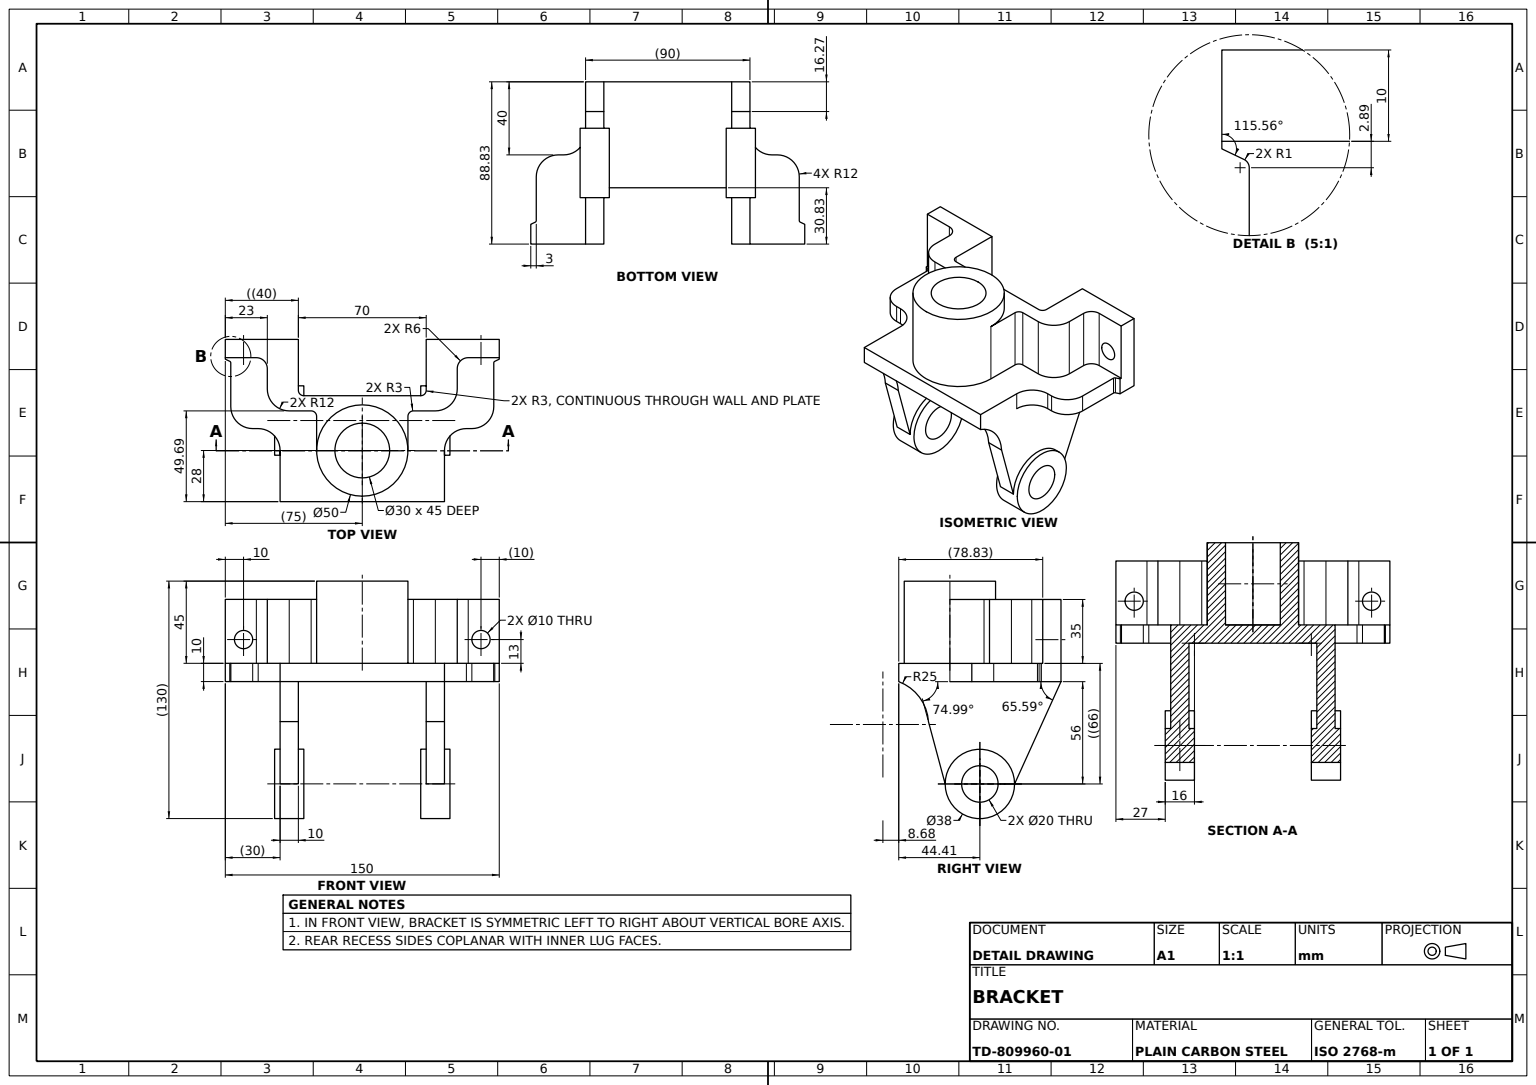
solid
v1 (-45,-61,-25.413573)
v2 (-45,-26.908854,-16.270281)
e1 v1 v2 LINE
v3 (-45,-5,0)
e2 v2 v3 CIRCLE(AX(P(-45,-28.443833,8.682552),D(1,0,0),D(0,0,1)),25)
v4 (-45,5,0)
e3 v4 v3 LINE
v5 (-45,5,-28)
e4 v5 v4 LINE
v6 (-45,-5,-28)
e5 v5 v6 LINE
v7 (-45,-5,-88.827146)
e6 v7 v6 LINE
v8 (-45,-61,-63.413573)
e7 v8 v7 LINE
e8 v1 v8 CIRCLE(AX(P(-45,-61,-44.413573),D(-1,0,0),D(0,0,1)),19)
face PLANE(AX(P(-45,5,0),D(1,0,0),D(0,0,-1))) rev [e1 e2 -e3 -e4 e5 -e6 -e7 -e8]
v9 (45,-5,-28)
v10 (57,-5,-40)
e9 v9 v10 CIRCLE(AX(P(57,-5,-28),D(0,-1,0),D(0,0,1)),12)
v11 (57,5,-40)
e10 v11 v10 LINE
v12 (45,5,-28)
e11 v12 v11 CIRCLE(AX(P(57,5,-28),D(0,-1,0),D(0,0,1)),12)
e12 v12 v9 LINE
face CYL(AX(P(57,5,-28),D(0,-1,0),D(0,0,-1)),12) rev [e9 -e10 -e11 e12]
v13 (35,-61,-63.413573)
v14 (32,-61,-63.413573)
e13 v13 v14 LINE
v15 (32,-61,-25.413573)
e14 v15 v14 CIRCLE(AX(P(32,-61,-44.413573),D(-1,0,0),D(0,0,1)),19)
v16 (35,-61,-25.413573)
e15 v16 v15 LINE
e16 v16 v13 CIRCLE(AX(P(35,-61,-44.413573),D(-1,0,0),D(0,0,1)),19)
face CYL(AX(P(48,-61,-44.413573),D(-1,0,0),D(0,0,1)),19) [e13 -e14 -e15 e16]
v17 (-32,-61,-34.413573)
v18 (-32,-61,-54.413573)
e17 v17 v18 CIRCLE(AX(P(-32,-61,-44.413573),D(-1,0,0),D(0,0,1)),10)
e18 v18 v17 CIRCLE(AX(P(-32,-61,-44.413573),D(-1,0,0),D(0,0,1)),10)
v19 (-32,-61,-63.413573)
v20 (-32,-61,-25.413573)
e19 v19 v20 CIRCLE(AX(P(-32,-61,-44.413573),D(-1,0,0),D(0,0,1)),19)
e20 v20 v19 CIRCLE(AX(P(-32,-61,-44.413573),D(-1,0,0),D(0,0,1)),19)
face PLANE(AX(P(-32,-61,-44.413573),D(-1,0,0),D(0,0,1))) rev [e17 e18] [-e19 -e20]
v21 (60,5,-40)
e21 v11 v21 LINE
v22 (60,-5,-40)
e22 v10 v22 LINE
e23 v21 v22 LINE
face PLANE(AX(P(57,5,-40),D(0,0,-1),D(-1,0,0))) rev [-e21 e10 e22 -e23]
v23 (-48,-61,-34.413573)
e24 v23 v17 LINE
v24 (-48,-61,-54.413573)
e25 v23 v24 CIRCLE(AX(P(-48,-61,-44.413573),D(-1,0,0),D(0,0,1)),10)
e26 v24 v18 LINE
face CYL(AX(P(-48,-61,-44.413573),D(1,0,0),D(0,0,-1)),10) rev [-e24 e25 e26 -e17]
v25 (35,-5,-61)
v26 (35,-5,0)
e27 v25 v26 LINE
v27 (-35,-5,0)
e28 v27 v26 LINE
v28 (-35,-5,-61)
e29 v28 v27 LINE
v29 (-32,-5,-58)
e30 v29 v28 CIRCLE(AX(P(-32,-5,-61),D(0,-1,0),D(0,0,1)),3)
v30 (32,-5,-58)
e31 v30 v29 LINE
e32 v25 v30 CIRCLE(AX(P(32,-5,-61),D(0,-1,0),D(0,0,1)),3)
face PLANE(AX(P(-57,-5,-28),D(0,-1,0),D(0,0,-1))) [e27 -e28 -e29 -e30 -e31 -e32]
v31 (-28,40,-49.686128)
v32 (-28,5,-49.686128)
e33 v31 v32 LINE
v33 (-25,5,-46.686128)
e34 v32 v33 CIRCLE(AX(P(-28,5,-46.686128),D(0,-1,0),D(0,0,1)),3)
v34 (-25,40,-46.686128)
e35 v34 v33 LINE
e36 v31 v34 CIRCLE(AX(P(-28,40,-46.686128),D(0,-1,0),D(0,0,1)),3)
face CYL(AX(P(-28,40,-46.686128),D(0,-1,0),D(0,0,-1)),3) rev [e33 e34 -e35 -e36]
v35 (-70,18,-78.827146)
v36 (-70,18,-88.827146)
e37 v35 v36 LINE
v37 (-60,18,-88.827146)
e38 v36 v37 CIRCLE(AX(P(-65,18,-88.827146),D(0,0,-1),D(-1,0,0)),5)
v38 (-60,18,-78.827146)
e39 v38 v37 LINE
e40 v35 v38 CIRCLE(AX(P(-65,18,-78.827146),D(0,0,-1),D(-1,0,0)),5)
face CYL(AX(P(-65,18,-66.327146),D(0,0,-1),D(-1,0,0)),5) rev [e37 e38 -e39 -e40]
v39 (52,40,-61.686128)
v40 (52,5,-61.686128)
e41 v39 v40 LINE
v41 (52,5,-72.827146)
e42 v41 v40 LINE
v42 (52,40,-72.827146)
e43 v42 v41 LINE
e44 v42 v39 LINE
face PLANE(AX(P(52,40,0),D(1,0,0),D(0,0,-1))) [e41 -e42 -e43 e44]
e45 v24 v23 CIRCLE(AX(P(-48,-61,-44.413573),D(-1,0,0),D(0,0,1)),10)
v43 (-48,-61,-63.413573)
v44 (-48,-61,-25.413573)
e46 v43 v44 CIRCLE(AX(P(-48,-61,-44.413573),D(-1,0,0),D(0,0,1)),19)
e47 v44 v43 CIRCLE(AX(P(-48,-61,-44.413573),D(-1,0,0),D(0,0,1)),19)
face PLANE(AX(P(-48,-61,-44.413573),D(-1,0,0),D(0,0,1))) [-e45 -e25] [e46 e47]
v45 (0,50,-43)
v46 (0,50,-13)
e48 v45 v46 CIRCLE(AX(P(0,50,-28),D(0,1,0),D(0,0,1)),15)
v47 (0,5,-13)
e49 v46 v47 LINE
v48 (0,5,-43)
e50 v48 v47 CIRCLE(AX(P(0,5,-28),D(0,1,0),D(0,0,1)),15)
e51 v45 v48 LINE
face CYL(AX(P(0,50,-28),D(0,-1,0),D(0,0,-1)),15) rev [e48 e49 -e50 -e51]
v49 (60,18,-88.827146)
v50 (70,18,-88.827146)
e52 v49 v50 CIRCLE(AX(P(65,18,-88.827146),D(0,0,-1),D(-1,0,0)),5)
v51 (70,18,-78.827146)
e53 v51 v50 LINE
v52 (60,18,-78.827146)
e54 v51 v52 CIRCLE(AX(P(65,18,-78.827146),D(0,0,1),D(1,0,0)),5)
e55 v52 v49 LINE
face CYL(AX(P(65,18,-66.327146),D(0,0,-1),D(-1,0,0)),5) rev [e52 -e53 e54 e55]
v53 (75,-5,-88.827146)
v54 (45,-5,-88.827146)
e56 v53 v54 LINE
v55 (35,-5,-88.827146)
e57 v55 v54 LINE
v56 (35,40,-88.827146)
e58 v55 v56 LINE
v57 (75,40,-88.827146)
e59 v57 v56 LINE
e60 v53 v57 LINE
e61 v50 v49 CIRCLE(AX(P(65,18,-88.827146),D(0,0,-1),D(-1,0,0)),5)
face PLANE(AX(P(35,-5,-88.827146),D(0,0,-1),D(-1,0,0))) [e56 -e57 e58 -e59 -e60] [-e61 -e52]
e62 v14 v15 CIRCLE(AX(P(32,-61,-44.413573),D(-1,0,0),D(0,0,1)),19)
v58 (45,-61,-63.413573)
e63 v13 v58 LINE
v59 (48,-61,-63.413573)
e64 v59 v58 LINE
v60 (48,-61,-25.413573)
e65 v59 v60 CIRCLE(AX(P(48,-61,-44.413573),D(-1,0,0),D(0,0,1)),19)
v61 (45,-61,-25.413573)
e66 v60 v61 LINE
e67 v16 v61 LINE
face CYL(AX(P(48,-61,-44.413573),D(-1,0,0),D(0,0,1)),19) [e15 -e62 -e13 e63 -e64 e65 e66 -e67]
e68 v58 v54 LINE
e69 v13 v55 LINE
face PLANE(AX(P(35,-34.280712,-75.539155),D(0,-0.413250701,-0.910617295),D(0,0.910617295,-0.413250701))) [-e68 -e63 e69 e57]
v62 (-72,5,-52)
v63 (-60,5,-40)
e70 v62 v63 CIRCLE(AX(P(-60,5,-52),D(0,1,0),D(0,0,-1)),12)
v64 (-72,-5,-52)
e71 v62 v64 LINE
v65 (-60,-5,-40)
e72 v64 v65 CIRCLE(AX(P(-60,-5,-52),D(0,1,0),D(0,0,-1)),12)
e73 v63 v65 LINE
face CYL(AX(P(-60,5,-52),D(0,-1,0),D(0,0,-1)),12) [-e70 e71 e72 -e73]
v66 (40,40,-49.686128)
v67 (40,5,-49.686128)
e74 v66 v67 LINE
e75 v40 v67 CIRCLE(AX(P(40,5,-61.686128),D(0,-1,0),D(0,0,1)),12)
e76 v39 v66 CIRCLE(AX(P(40,40,-61.686128),D(0,-1,0),D(0,0,1)),12)
face CYL(AX(P(40,40,-61.686128),D(0,-1,0),D(0,0,-1)),12) [e74 -e75 -e41 e76]
v68 (32,40,-58)
v69 (-32,40,-58)
e77 v68 v69 LINE
e78 v68 v30 LINE
e79 v69 v29 LINE
face PLANE(AX(P(-32,5,-58),D(0,0,1),D(1,0,0))) rev [-e77 e78 e31 -e79]
v70 (45,5,0)
e80 v70 v12 LINE
v71 (45,-5,0)
e81 v70 v71 LINE
v72 (45,-26.908854,-16.270281)
e82 v72 v71 CIRCLE(AX(P(45,-28.443833,8.682552),D(1,0,0),D(0,0,1)),25)
e83 v61 v72 LINE
e84 v61 v58 CIRCLE(AX(P(45,-61,-44.413573),D(-1,0,0),D(0,0,1)),19)
e85 v54 v9 LINE
face PLANE(AX(P(45,5,0),D(-1,0,0),D(0,0,1))) rev [-e80 e81 -e82 -e83 e84 e68 e85 -e12]
v73 (35,40,-61)
e86 v73 v68 CIRCLE(AX(P(32,40,-61),D(0,-1,0),D(0,0,1)),3)
e87 v73 v25 LINE
face CYL(AX(P(32,5,-61),D(0,-1,0),D(0,0,-1)),3) rev [e32 -e78 -e86 e87]
v74 (25,40,-28)
v75 (25,40,-46.686128)
e88 v74 v75 LINE
v76 (25,5,-28)
e89 v74 v76 LINE
v77 (25,5,-46.686128)
e90 v76 v77 LINE
e91 v75 v77 LINE
face PLANE(AX(P(25,40,0),D(-1,0,0),D(0,0,1))) rev [-e88 e89 e90 -e91]
e92 v44 v1 LINE
e93 v43 v8 LINE
face CYL(AX(P(-48,-61,-44.413573),D(1,0,0),D(0,0,-1)),19) [e92 e8 -e93 -e47]
v78 (72,5,-52)
e94 v21 v78 CIRCLE(AX(P(60,5,-52),D(0,1,0),D(0,0,-1)),12)
v79 (72,-5,-52)
e95 v22 v79 CIRCLE(AX(P(60,-5,-52),D(0,1,0),D(0,0,-1)),12)
e96 v78 v79 LINE
face CYL(AX(P(60,5,-52),D(0,-1,0),D(0,0,-1)),12) [-e94 e23 e95 -e96]
v80 (-52,40,-72.827146)
v81 (-58,40,-78.827146)
e97 v80 v81 CIRCLE(AX(P(-58,40,-72.827146),D(0,1,0),D(0,0,1)),6)
v82 (-58,5,-78.827146)
e98 v81 v82 LINE
v83 (-52,5,-72.827146)
e99 v83 v82 CIRCLE(AX(P(-58,5,-72.827146),D(0,1,0),D(0,0,1)),6)
e100 v80 v83 LINE
face CYL(AX(P(-58,40,-72.827146),D(0,-1,0),D(0,0,-1)),6) rev [e97 e98 -e99 -e100]
e101 v3 v27 LINE
e102 v26 v71 LINE
e103 v4 v70 LINE
face PLANE(AX(P(-45,5,0),D(0,0,-1),D(-1,0,0))) rev [e101 e28 e102 -e81 -e103 e3]
v84 (-35,-5,-88.827146)
v85 (-35,40,-88.827146)
e104 v84 v85 LINE
e105 v84 v7 LINE
v86 (-75,-5,-88.827146)
e106 v7 v86 LINE
v87 (-75,40,-88.827146)
e107 v86 v87 LINE
e108 v85 v87 LINE
e109 v37 v36 CIRCLE(AX(P(-65,18,-88.827146),D(0,0,-1),D(-1,0,0)),5)
face PLANE(AX(P(-75,-5,-88.827146),D(0,0,-1),D(-1,0,0))) [-e104 e105 e106 e107 -e108] [-e38 -e109]
v88 (72,5,-75.935047)
v89 (72,-5,-75.935047)
e110 v88 v89 LINE
v90 (72.56856,-5,-76.837188)
e111 v89 v90 CIRCLE(AX(P(73,-5,-75.935047),D(0,-1,0),D(0,0,1)),1)
v91 (72.56856,5,-76.837188)
e112 v91 v90 LINE
e113 v88 v91 CIRCLE(AX(P(73,5,-75.935047),D(0,-1,0),D(0,0,1)),1)
face CYL(AX(P(73,5,-75.935047),D(0,-1,0),D(0,0,-1)),1) rev [e110 e111 -e112 -e113]
face CYL(AX(P(-48,-61,-44.413573),D(1,0,0),D(0,0,-1)),10) rev [-e18 -e26 e45 e24]
v92 (-72.56856,5,-76.837188)
v93 (-72.56856,-5,-76.837188)
e114 v92 v93 LINE
v94 (-72,-5,-75.935047)
e115 v93 v94 CIRCLE(AX(P(-73,-5,-75.935047),D(0,-1,0),D(0,0,1)),1)
v95 (-72,5,-75.935047)
e116 v95 v94 LINE
e117 v92 v95 CIRCLE(AX(P(-73,5,-75.935047),D(0,-1,0),D(0,0,1)),1)
face CYL(AX(P(-73,5,-75.935047),D(0,-1,0),D(0,0,-1)),1) rev [e114 e115 -e116 -e117]
e118 v60 v59 CIRCLE(AX(P(48,-61,-44.413573),D(-1,0,0),D(0,0,1)),19)
face CYL(AX(P(48,-61,-44.413573),D(-1,0,0),D(0,0,1)),19) [e118 e64 -e84 -e66]
e119 v38 v35 CIRCLE(AX(P(-65,18,-78.827146),D(0,0,-1),D(-1,0,0)),5)
v96 (-75,5,-78.827146)
e120 v96 v82 LINE
v97 (-75,40,-78.827146)
e121 v97 v81 LINE
e122 v97 v96 LINE
face PLANE(AX(P(0,40,-78.827146),D(0,0,-1),D(-1,0,0))) rev [e119 e40] [e120 -e98 -e121 e122]
face CYL(AX(P(-65,18,-66.327146),D(0,0,-1),D(-1,0,0)),5) rev [e109 -e37 -e119 e39]
v98 (-25,5,-28)
e123 v98 v33 LINE
v99 (-25,40,-28)
e124 v99 v98 LINE
e125 v99 v34 LINE
face PLANE(AX(P(-25,40,0),D(-1,0,0),D(0,0,1))) [-e123 -e124 e125 e35]
v100 (58,40,-78.827146)
v101 (58,5,-78.827146)
e126 v100 v101 LINE
v102 (75,5,-78.827146)
e127 v102 v101 LINE
v103 (75,40,-78.827146)
e128 v103 v102 LINE
e129 v103 v100 LINE
e130 v52 v51 CIRCLE(AX(P(65,18,-78.827146),D(0,0,1),D(1,0,0)),5)
face PLANE(AX(P(0,40,-78.827146),D(0,0,1),D(1,0,0))) [e126 -e127 -e128 e129] [-e130 -e54]
v104 (-35,-26.908854,-16.270281)
e131 v104 v2 LINE
e132 v104 v27 CIRCLE(AX(P(-35,-28.443833,8.682552),D(1,0,0),D(0,0,1)),25)
face CYL(AX(P(-35,-28.443833,8.682552),D(-1,0,0),D(0,0,1)),25) rev [-e2 -e131 e132 -e101]
v105 (-57,5,-40)
e133 v105 v5 CIRCLE(AX(P(-57,5,-28),D(0,-1,0),D(0,0,-1)),12)
v106 (-57,-5,-40)
e134 v105 v106 LINE
e135 v106 v6 CIRCLE(AX(P(-57,-5,-28),D(0,-1,0),D(0,0,-1)),12)
face CYL(AX(P(-57,5,-28),D(0,-1,0),D(0,0,-1)),12) rev [-e133 e134 e135 -e5]
v107 (0,50,-3)
v108 (0,50,-53)
e136 v107 v108 CIRCLE(AX(P(0,50,-28),D(0,1,0),D(0,0,1)),25)
e137 v108 v107 CIRCLE(AX(P(0,50,-28),D(0,1,0),D(0,0,1)),25)
e138 v46 v45 CIRCLE(AX(P(0,50,-28),D(0,1,0),D(0,0,1)),15)
face PLANE(AX(P(0,50,0),D(0,1,0),D(0,0,1))) [e136 e137] [-e48 -e138]
v109 (28,40,-49.686128)
e139 v109 v66 LINE
v110 (28,5,-49.686128)
e140 v109 v110 LINE
e141 v110 v67 LINE
face PLANE(AX(P(0,40,-49.686128),D(0,0,-1),D(-1,0,0))) rev [-e139 e140 e141 -e74]
e142 v47 v48 CIRCLE(AX(P(0,5,-28),D(0,1,0),D(0,0,1)),15)
face PLANE(AX(P(-57,5,-28),D(0,-1,0),D(0,0,-1))) rev [e142 e50]
e143 v65 v106 LINE
e144 v63 v105 LINE
face PLANE(AX(P(-57,5,-40),D(0,0,-1),D(-1,0,0))) rev [e73 e143 -e134 -e144]
v111 (-35,-61,-63.413573)
e145 v111 v84 LINE
e146 v111 v8 LINE
face PLANE(AX(P(-35,-34.280712,-75.539155),D(0,0.413250701,0.910617295),D(0,-0.910617295,0.413250701))) rev [-e105 -e145 e146 e7]
v112 (-75,5,-78)
e147 v112 v92 LINE
v113 (-75,-5,-78)
e148 v112 v113 LINE
e149 v113 v93 LINE
face PLANE(AX(P(-75,5,-78),D(0.431440099,0,-0.902141586),D(-0.902141586,0,-0.431440099))) rev [-e114 -e147 e148 e149]
v114 (-40,40,-49.686128)
v115 (-40,5,-49.686128)
e150 v114 v115 LINE
e151 v32 v115 LINE
e152 v31 v114 LINE
face PLANE(AX(P(0,40,-49.686128),D(0,0,1),D(1,0,0))) [e150 -e151 -e33 e152]
face CYL(AX(P(0,50,-28),D(0,-1,0),D(0,0,-1)),15) rev [e138 e51 -e142 -e49]
v116 (48,-61,-34.413573)
v117 (48,-61,-54.413573)
e153 v116 v117 CIRCLE(AX(P(48,-61,-44.413573),D(-1,0,0),D(0,0,1)),10)
v118 (32,-61,-34.413573)
e154 v116 v118 LINE
v119 (32,-61,-54.413573)
e155 v118 v119 CIRCLE(AX(P(32,-61,-44.413573),D(-1,0,0),D(0,0,1)),10)
e156 v117 v119 LINE
face CYL(AX(P(48,-61,-44.413573),D(-1,0,0),D(0,0,1)),10) rev [-e153 e154 e155 -e156]
v120 (35,-26.908854,-16.270281)
e157 v120 v26 CIRCLE(AX(P(35,-28.443833,8.682552),D(1,0,0),D(0,0,1)),25)
e158 v120 v72 LINE
face CYL(AX(P(35,-28.443833,8.682552),D(1,0,0),D(0,0,-1)),25) rev [-e102 -e157 e158 e82]
e159 v119 v118 CIRCLE(AX(P(32,-61,-44.413573),D(-1,0,0),D(0,0,1)),10)
face PLANE(AX(P(32,-61,-44.413573),D(1,0,0),D(0,0,1))) rev [e62 e14] [-e159 -e155]
v121 (-35,-61,-25.413573)
e160 v121 v1 LINE
e161 v121 v104 LINE
face PLANE(AX(P(-35,2.265167,-8.445768),D(0,-0.259046303,0.965864904),D(0,-0.965864904,-0.259046303))) [e131 -e1 -e160 e161]
e162 v94 v64 LINE
e163 v86 v113 LINE
face PLANE(AX(P(-57,-5,-28),D(0,-1,0),D(0,0,-1))) [-e72 -e162 -e115 -e149 -e163 -e106 e6 -e135 -e143]
e164 v56 v73 LINE
e165 v16 v120 LINE
face PLANE(AX(P(35,5,-61),D(1,0,0),D(0,0,-1))) rev [-e164 -e58 -e69 -e16 e165 e157 -e27 -e87]
e166 v96 v112 LINE
e167 v87 v97 LINE
face PLANE(AX(P(-75,-5,-78),D(-1,0,0),D(0,0,1))) [-e107 e163 -e148 -e166 -e122 -e167]
e168 v121 v111 CIRCLE(AX(P(-35,-61,-44.413573),D(-1,0,0),D(0,0,1)),19)
v122 (-35,40,-61)
e169 v122 v85 LINE
e170 v122 v28 LINE
face PLANE(AX(P(-35,5,-78),D(-1,0,0),D(0,0,1))) rev [e29 -e132 -e161 e168 e145 e104 -e169 e170]
e171 v103 v57 LINE
v123 (75,5,-78)
e172 v123 v102 LINE
v124 (75,-5,-78)
e173 v123 v124 LINE
e174 v124 v53 LINE
face PLANE(AX(P(75,-5,-88.827146),D(1,0,0),D(0,0,-1))) [e60 -e171 e128 -e172 e173 e174]
v125 (0,40,-53)
e175 v108 v125 LINE
e176 v125 v99 CIRCLE(AX(P(0,40,-28),D(0,1,0),D(0,0,1)),25)
v126 (0,5,-3)
e177 v98 v126 CIRCLE(AX(P(0,5,-28),D(0,1,0),D(0,0,1)),25)
e178 v107 v126 LINE
face CYL(AX(P(0,50,-28),D(0,-1,0),D(0,0,-1)),25) [e175 e176 e124 e177 -e178 -e137]
e179 v117 v116 CIRCLE(AX(P(48,-61,-44.413573),D(-1,0,0),D(0,0,1)),10)
face PLANE(AX(P(48,-61,-44.413573),D(1,0,0),D(0,0,1))) [e179 e153] [-e118 -e65]
face PLANE(AX(P(35,2.265167,-8.445768),D(0,0.259046303,-0.965864904),D(0,0.965864904,0.259046303))) rev [e83 -e158 -e165 e67]
v127 (-52,40,-61.686128)
v128 (-52,5,-61.686128)
e180 v127 v128 LINE
e181 v80 v127 LINE
e182 v83 v128 LINE
face PLANE(AX(P(-52,40,0),D(1,0,0),D(0,0,-1))) rev [-e180 -e181 e100 e182]
e183 v69 v122 CIRCLE(AX(P(-32,40,-61),D(0,-1,0),D(0,0,1)),3)
face CYL(AX(P(-32,5,-61),D(0,-1,0),D(0,0,-1)),3) rev [e30 -e170 -e183 e79]
face CYL(AX(P(48,-61,-44.413573),D(-1,0,0),D(0,0,1)),10) rev [-e179 e156 e159 -e154]
e184 v110 v77 CIRCLE(AX(P(28,5,-46.686128),D(0,1,0),D(0,0,1)),3)
e185 v109 v75 CIRCLE(AX(P(28,40,-46.686128),D(0,1,0),D(0,0,1)),3)
face CYL(AX(P(28,40,-46.686128),D(0,-1,0),D(0,0,-1)),3) rev [e91 -e184 -e140 e185]
e186 v95 v62 LINE
face PLANE(AX(P(-72,5,-52),D(1,0,0),D(0,0,-1))) rev [e116 e162 -e71 -e186]
e187 v74 v125 CIRCLE(AX(P(0,40,-28),D(0,1,0),D(0,0,1)),25)
e188 v126 v76 CIRCLE(AX(P(0,5,-28),D(0,1,0),D(0,0,1)),25)
face CYL(AX(P(0,50,-28),D(0,-1,0),D(0,0,-1)),25) [e187 -e175 -e136 e178 e188 -e89]
e189 v79 v89 LINE
e190 v78 v88 LINE
face PLANE(AX(P(72,5,-52),D(-1,0,0),D(0,0,1))) rev [e189 -e110 -e190 e96]
e191 v121 v20 LINE
e192 v111 v19 LINE
face CYL(AX(P(-48,-61,-44.413573),D(1,0,0),D(0,0,-1)),19) [e19 -e191 e160 -e92 -e46 e93 -e146 e192]
e193 v114 v127 CIRCLE(AX(P(-40,40,-61.686128),D(0,-1,0),D(0,0,1)),12)
e194 v42 v100 CIRCLE(AX(P(58,40,-72.827146),D(0,-1,0),D(0,0,1)),6)
face PLANE(AX(P(0,40,0),D(0,1,0),D(0,0,1))) [e169 e108 e167 e121 -e97 e181 -e193 -e152 e36 -e125 -e176 -e187 e88 -e185 e139 -e76 -e44 e194 -e129 e171 e59 e164 e86 e77 e183]
e195 v90 v124 LINE
e196 v91 v123 LINE
face PLANE(AX(P(75,5,-78),D(-0.431440099,0,-0.902141586),D(-0.902141586,0,0.431440099))) rev [e195 -e173 -e196 e112]
face CYL(AX(P(-48,-61,-44.413573),D(1,0,0),D(0,0,-1)),19) [-e192 -e168 e191 e20]
e197 v41 v101 CIRCLE(AX(P(58,5,-72.827146),D(0,-1,0),D(0,0,1)),6)
e198 v115 v128 CIRCLE(AX(P(-40,5,-61.686128),D(0,-1,0),D(0,0,1)),12)
face PLANE(AX(P(-57,5,-28),D(0,-1,0),D(0,0,-1))) rev [e186 e70 e144 e133 e4 e103 e80 e11 e21 e94 e190 e113 e196 e172 e127 -e197 e42 e75 -e141 e184 -e90 -e188 -e177 e123 -e34 e151 e198 -e182 e99 -e120 e166 e147 e117]
face CYL(AX(P(65,18,-66.327146),D(0,0,-1),D(-1,0,0)),5) rev [-e55 e130 e53 e61]
face CYL(AX(P(-40,40,-61.686128),D(0,-1,0),D(0,0,-1)),12) [e180 -e198 -e150 e193]
face PLANE(AX(P(-57,-5,-28),D(0,-1,0),D(0,0,-1))) [-e189 -e95 -e22 -e9 -e85 -e56 -e174 -e195 -e111]
face CYL(AX(P(58,40,-72.827146),D(0,-1,0),D(0,0,-1)),6) rev [-e126 -e194 e43 e197]
